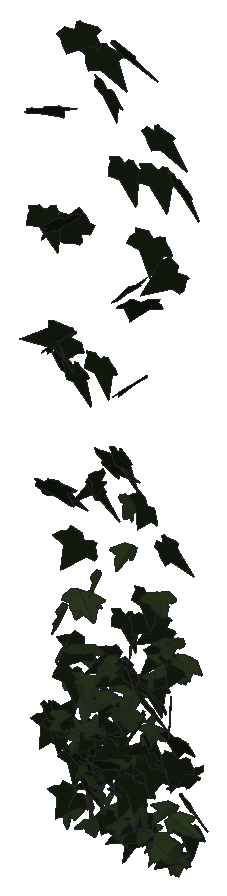
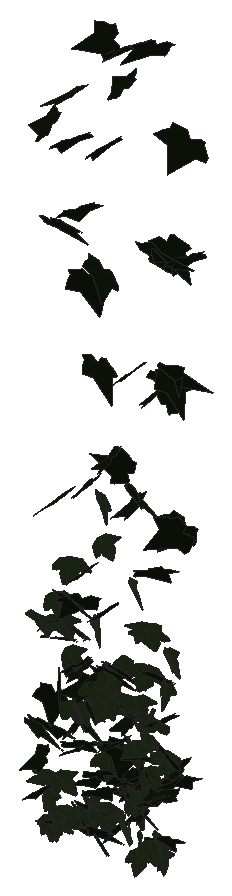
# SketchUp Ruby script. Lengths in inches.
U = 1.inch
M = Sketchup.active_model
def pt(a) = Geom::Point3d.new(a.map { |v| v * U })
def face(e, loops, mat)
  f = e.add_face(loops[0].map { |a| pt(a) })
  loops[1..].each { |l| e.add_face(l.map { |a| pt(a) }).erase! }
  f.material = f.back_material = mat if mat
  f
end
# faces: each face lists its corners as indices into pts; further lists are holes
def faces(e, pts, list, mat = nil) = list.each { |f| face(e, (f[0].is_a?(Array) ? f : [f]).map { |l| l.map { |i| pts[i] } }, mat) }
# xy, xz, yz: faces in a plane at the given z, y or x. An outline is a flat list of corners, or four numbers for a rectangle; further outlines are holes
def ring(l) = l.size == 4 ? [[l[0], l[1]], [l[2], l[1]], [l[2], l[3]], [l[0], l[3]]] : l.each_slice(2).to_a
def flat(e, list, mat, &to3) = list.each { |f| face(e, (f[0].is_a?(Array) ? f : [f]).map { |l| ring(l).map { |u, v| to3.(u, v) } }, mat) }
def xy(e, z, list, mat = nil) = flat(e, list, mat) { |x, y| [x, y, z] }
def xz(e, y, list, mat = nil) = flat(e, list, mat) { |x, z| [x, y, z] }
def yz(e, x, list, mat = nil) = flat(e, list, mat) { |y, z| [x, y, z] }
def lines(e, pts, list) = list.each { |a, b| e.add_line(pt(pts[a]), pt(pts[b])) }
# prism: a flat outline (further loops are holes) pulled along v
def prism(e, loops, v, mat = nil)
  f = face(e, loops, mat); d = Geom::Vector3d.new(v.map { |x| x * U })
  f.pushpull(f.normal.samedirection?(d) ? d.length : -d.length)
end
def box(e, o, s, mat = nil) = prism(e, [[o, [o[0] + s[0], o[1], o[2]], [o[0] + s[0], o[1] + s[1], o[2]], [o[0], o[1] + s[1], o[2]]]], [0, 0, s[2]], mat)
def at(x, y, z, deg = 0) = Geom::Transformation.translation(pt([x, y, z])) * Geom::Transformation.rotation(ORIGIN, Z_AXIS, deg.degrees)
def axes(o, x, y, z) = Geom::Transformation.new([*x, 0, *y, 0, *z, 0, *pt(o).to_a, 1])
def part(name) = M.definitions.add(name)
# library, detail: a bought-in or finely detailed component or shape, given as its bounding box
def library(name, o, s) = part(name).tap { |d| box(d.entities, o, s) }
def detail(e, o, s) = box(e.add_group.entities, o, s)
def put(e, d, t, mat = nil) = e.add_instance(d, t).tap { |i| i.material = mat if mat }
def group(e, t, mat = nil) = e.add_group.tap { |g| g.transformation = t; g.material = mat if mat }.entities
root = M.entities
M.materials.add("1026 AP 7946 SUNNY SIDE UP").color = [254, 231, 186]
M.materials.add("efeu1").color = [18, 25, 13]
M.materials.add("efeu2").color = [43, 57, 29]
c1 = part("ivyleaf_9")
p = [[1.54,2.16,1.25],[1.36,2.04,1.19],[-0.21,0.99,0.68],[-0.71,1.11,0.82],[-0.85,0.86,0.67],[-0.8,0.17,0.21],
  [-0.9,-0.01,0.1],[-0.67,-0.16,-0.02],[-0.08,-0.08,-0.05],[-0.03,-0.6,-0.4],[0.65,-0.88,-0.66],[0.83,-0.6,-0.49],
  [1.29,-0.42,-0.43],[1.8125,-0.07,-0.26],[1.21,0.44,0.15]]
faces(c1.entities,p,[[0,1,2,3,4,5,6,7,8,9,10,11,12,13,14]],"efeu1")
c2 = part("ivyleaf_10")
p = [[0,0.5,-0.03],[-0.0625,2.02,-0.43],[-0.19,2.01,-0.46],[-0.54,1.05,-0.29],[-0.52,0.625,-0.18],[-0.83,0.76,-0.28],
  [-1.16,0.64,-0.33],[-1.15,0.33,-0.24],[-0.77,-0.39,0.02],[-0.3,-0.51,0.16],[0.04,-0.48,0.23],[-0.02,2.01,-0.4375],
  [-0.06,2.01,-0.43],[0.04,-0.49,0.23],[0.67,-0.49,0.14],[1.38,0.36,-0.2],[1.375,0.51,-0.24],[0.81,0.65,-0.19],
  [0.62,0.59,-0.15],[0.6,1.09,-0.28],[0.5,1.23,-0.31]]
faces(c2.entities,p,[[0,1,2,3,4,5,6,7,8,9,10],[11,12,0,13,14,15,16,17,18,19,20]],"efeu2")
put(root,c1,axes([140.27,212.33,315.16],[-0.05103,-0.41878,-0.14855],[0.02164,0.14117,-0.43188],[0.69488,-0.03515,0.00254]),"1026 AP 7946 SUNNY SIDE UP")
put(root,c1,axes([140.4375,211.97,319.57],[0.50058,0.35673,0.06426],[-0.02996,0.0968,-0.4854],[-0.56811,0.30923,0.08221]),"1026 AP 7946 SUNNY SIDE UP")
put(root,c1,axes([140.57,212.51,294.58],[-0.36705,-0.28376,0.04945],[-0.02292,-0.05214,-0.37818],[0.45238,-0.23288,0.02096]),"1026 AP 7946 SUNNY SIDE UP")
put(root,c1,axes([140.3,212.48,295.11],[0.31532,-0.31436,-0.0618],[-0.04224,0.05189,-0.38379],[0.50093,0.20226,0.00653]),"1026 AP 7946 SUNNY SIDE UP")
put(root,c1,axes([140.9,212.33,310.2],[-0.0672,0.44029,-0.05517],[0.00492,-0.05601,-0.45604],[-0.69789,-0.04279,0.0021]),"1026 AP 7946 SUNNY SIDE UP")
put(root,c1,axes([141.19,212.43,310.375],[-0.10965,-0.09175,-0.44165],[-0.41434,-0.3375,0.11673],[-0.54994,0.27258,0.00011]),"1026 AP 7946 SUNNY SIDE UP")
put(root,c1,axes([140.54,212.12,304.4],[0.60737,0.11779,-0.0227],[-0.01672,-0.04262,-0.41446],[-0.18788,0.38458,-0.03649]),"1026 AP 7946 SUNNY SIDE UP")
put(root,c1,axes([140.66,212.67,294.48],[-0.12026,-0.35836,0.0457],[-0.00253,-0.04709,-0.37768],[0.56819,-0.07606,0.00799]),"1026 AP 7946 SUNNY SIDE UP")
put(root,c1,axes([140.51,212.26,304.2],[0.63153,0.08305,0.10577],[0.17132,-0.02531,-0.42006],[-0.1163,0.41366,-0.04441]),"1026 AP 7946 SUNNY SIDE UP")
put(root,c1,axes([141.07,212.35,309.2],[0.26067,-0.24492,0.33514],[-0.16241,0.31599,0.29988],[-0.62117,-0.1854,0.06224]),"1026 AP 7946 SUNNY SIDE UP")
put(root,c2,axes([140.95,212.3,299.18],[0.16917,-0.36964,0.06288],[0.00554,-0.06468,-0.3967],[0.58962,0.10666,-0.01431]),"1026 AP 7946 SUNNY SIDE UP")
put(root,c2,axes([140.92,212.49,299.25],[0.31682,-0.31954,0.1033],[0.04111,-0.10376,-0.38837],[0.52586,0.20063,-0.03187]),"1026 AP 7946 SUNNY SIDE UP")
put(root,c1,axes([141.22,212.12,315.29],[-0.08166,0.39451,-0.22855],[-0.01903,-0.22668,-0.40955],[-0.71317,-0.03912,0.0371]),"1026 AP 7946 SUNNY SIDE UP")
put(root,c1,axes([141.66,212.4375,314.79],[-0.23021,0.14305,0.4165],[-0.53671,0.21835,-0.20607],[-0.40626,-0.36953,0.03623]),"1026 AP 7946 SUNNY SIDE UP")
put(root,c1,axes([141,212.22,294.9],[-0.30917,0.27819,0.21651],[0.18946,-0.17027,0.34995],[0.51285,0.23061,0.00124]),"1026 AP 7946 SUNNY SIDE UP")
put(root,c2,axes([141.18,212.26,297.93],[0.00805,-0.35803,-0.18452],[0.06659,0.17658,-0.36551],[0.62452,-0.01421,0.04135]),"1026 AP 7946 SUNNY SIDE UP")
put(root,c2,axes([141.39,212.22,295.08],[0.47396,-0.01439,-0.23336],[-0.35019,0.05326,-0.30858],[0.06825,0.37322,0.03727]),"1026 AP 7946 SUNNY SIDE UP")
put(root,c2,axes([141.16,212.49,291.29],[-0.00569,-0.34874,0.06949],[0.12653,-0.06843,-0.3502],[0.54462,0.01226,0.08209]),"1026 AP 7946 SUNNY SIDE UP")
put(root,c1,axes([141.34,212.51,291.95],[-0.43317,-0.23152,0.01127],[0.01363,-0.0293,-0.36977],[0.3643,-0.2742,0.02723]),"1026 AP 7946 SUNNY SIDE UP")
put(root,c2,axes([141.32,212.64,292.03],[0.22658,-0.33741,-0.01255],[-0.00765,0.00908,-0.37792],[0.53074,0.14418,-0.00009]),"1026 AP 7946 SUNNY SIDE UP")
put(root,c2,axes([141.0625,212.53,295.0625],[0.30439,-0.2512,0.21366],[0.34212,-0.0819,-0.30976],[0.38312,0.27271,0.10687]),"1026 AP 7946 SUNNY SIDE UP")
put(root,c1,axes([141.15,212.66,296.77],[-0.07297,-0.37912,-0.02091],[0.03044,0.01589,-0.39298],[0.59603,-0.04723,0.01751]),"1026 AP 7946 SUNNY SIDE UP")
put(root,c1,axes([141.13,212.63,293.65],[-0.13427,-0.28959,0.21536],[0.31555,-0.21809,-0.22629],[0.46639,0.06418,0.2151]),"1026 AP 7946 SUNNY SIDE UP")
put(root,c2,axes([141.58,212.65,291.67],[-0.35002,-0.27086,0.09031],[-0.00772,-0.1095,-0.35581],[0.44834,-0.21335,0.06438]),"1026 AP 7946 SUNNY SIDE UP")
put(root,c1,axes([141.54,212.64,293.45],[-0.20851,-0.3427,0.05843],[0.0096,-0.06507,-0.37777],[0.54661,-0.12958,0.02892]),"1026 AP 7946 SUNNY SIDE UP")
put(root,c2,axes([141.75,212.54,294.4],[-0.15602,-0.31038,0.17899],[-0.03212,-0.17693,-0.33527],[0.55974,-0.09667,0.03065]),"1026 AP 7946 SUNNY SIDE UP")
put(root,c1,axes([141.79,212.46,302.34],[-0.46187,-0.29028,0.06023],[-0.03319,-0.06393,-0.42467],[0.46495,-0.29293,0.02952]),"1026 AP 7946 SUNNY SIDE UP")
put(root,c2,axes([141.38,212.6,296.58],[0.49346,0.11332,0.21476],[0.32955,0.02739,-0.34127],[-0.173,0.3754,-0.03752]),"1026 AP 7946 SUNNY SIDE UP")
put(root,c1,axes([141.89,212.37,298.23],[-0.59094,-0.10328,-0.02932],[0.06474,-0.04568,-0.3978],[0.15526,-0.37407,0.05429]),"1026 AP 7946 SUNNY SIDE UP")
put(root,c2,axes([141.64,212.61,300],[0.5861,0.1408,-0.03835],[-0.03035,-0.05581,-0.40816],[-0.22731,0.3705,-0.04438]),"1026 AP 7946 SUNNY SIDE UP")
put(root,c2,axes([141.82,212.27,296.57],[-0.20291,0.34701,0.07481],[-0.05385,0.06261,-0.3809],[-0.55422,-0.13313,0.00962]),"1026 AP 7946 SUNNY SIDE UP")
put(root,c1,axes([141.57,212.27,309.35],[0.23878,-0.40183,-0.02146],[-0.02673,0.0134,-0.44231],[0.63195,0.1524,-0.0106]),"1026 AP 7946 SUNNY SIDE UP")
put(root,c1,axes([141.6875,212.25,323.01],[0.1133,-0.29523,-0.36052],[0.0929,0.35565,-0.29591],[0.71188,0.00057,0.09599]),"1026 AP 7946 SUNNY SIDE UP")
put(root,c2,axes([141.92,212.48,295.92],[0.51465,-0.16428,0.11376],[0.14985,-0.05829,-0.3775],[0.27373,0.34078,-0.00722]),"1026 AP 7946 SUNNY SIDE UP")
put(root,c1,axes([142.32,212.25,294.15],[-0.01414,0.02527,0.41183],[-0.09221,0.39533,-0.0248],[-0.62283,-0.0591,-0.00568]),"1026 AP 7946 SUNNY SIDE UP")
put(root,c2,axes([141.88,212.375,300.09],[0.36462,0.31007,0.11714],[0.15168,0.06706,-0.39679],[-0.49567,0.24861,-0.03525]),"1026 AP 7946 SUNNY SIDE UP")
put(root,c2,axes([142.08,212.22,298.21],[-0.52991,-0.18021,-0.07781],[0.13377,-0.002,-0.39143],[0.27591,-0.34514,0.04032]),"1026 AP 7946 SUNNY SIDE UP")
put(root,c2,axes([142.14,212.5625,291.1],[-0.27695,-0.30984,-0.07147],[0.07114,0.052,-0.3666],[0.49356,-0.18135,0.01274]),"1026 AP 7946 SUNNY SIDE UP")
put(root,c2,axes([142.1,212.21,293.52],[0.00377,-0.33346,-0.1644],[0.09303,0.15599,-0.338],[0.57249,-0.02315,0.05601]),"1026 AP 7946 SUNNY SIDE UP")
put(root,c2,axes([142.15,212.5,291.67],[-0.22791,0.32533,-0.0754],[-0.05562,-0.09631,-0.36032],[-0.52203,-0.13177,0.07131]),"1026 AP 7946 SUNNY SIDE UP")
put(root,c1,axes([141.96,212.41,294.07],[0.26741,-0.32817,-0.01308],[-0.02667,0.0034,-0.3805],[0.5156,0.17038,-0.0129]),"1026 AP 7946 SUNNY SIDE UP")
put(root,c1,axes([142.32,212.6,294.83],[-0.40803,-0.26374,0.07918],[0.02976,-0.12457,-0.36809],[0.4316,-0.24075,0.10024]),"1026 AP 7946 SUNNY SIDE UP")
put(root,c1,axes([142.59,212.45,293.04],[-0.45307,0.227,-0.02686],[0.00491,-0.0401,-0.3769],[-0.35949,-0.28664,0.0287]),"1026 AP 7946 SUNNY SIDE UP")
put(root,c1,axes([142.03,212.32,292.83],[0.40398,-0.30202,-0.04531],[-0.07259,0.01612,-0.40761],[0.474,0.25987,-0.0238]),"1026 AP 7946 SUNNY SIDE UP")
put(root,c2,axes([142.61,212.21,292.79],[-0.47002,0.12116,0.23185],[-0.35052,0.04369,-0.33],[-0.19467,-0.3712,0.0344]),"1026 AP 7946 SUNNY SIDE UP")
put(root,c2,axes([142.39,212.41,296.95],[-0.30169,-0.31803,0.106],[0.0274,-0.12999,-0.37464],[0.52576,-0.17572,0.08035]),"1026 AP 7946 SUNNY SIDE UP")
put(root,c2,axes([142.4,212.55,293.3],[-0.52141,0.15638,-0.01607],[0.00175,-0.03614,-0.37645],[-0.24725,-0.33004,0.03122]),"1026 AP 7946 SUNNY SIDE UP")
put(root,c2,axes([142.47,212.37,295.125],[-0.29512,-0.33445,0.07364],[0.01329,-0.08818,-0.39229],[0.53823,-0.1812,0.05006]),"1026 AP 7946 SUNNY SIDE UP")
put(root,c1,axes([142.71,212.3125,305.17],[-0.5278,0.19491,-0.14126],[0.14523,-0.11399,-0.39732],[-0.34652,-0.34465,0.04864]),"1026 AP 7946 SUNNY SIDE UP")
put(root,c1,axes([142.48,212.73,293.9375],[-0.20009,-0.33888,0.08114],[-0.0045,-0.08488,-0.37241],[0.54774,-0.12449,0.02658]),"1026 AP 7946 SUNNY SIDE UP")
put(root,c2,axes([142.41,212.71,293.64],[0.41764,-0.21258,0.15038],[0.17783,-0.09422,-0.35102],[0.3656,0.28867,-0.00105]),"1026 AP 7946 SUNNY SIDE UP")
put(root,c2,axes([142.3,212.55,295.09],[-0.05262,-0.06988,-0.37603],[0.3321,-0.30466,0.0384],[-0.48008,-0.20309,0.06778]),"1026 AP 7946 SUNNY SIDE UP")
put(root,c2,axes([142.65,212.23,301.29],[0.30959,-0.34036,0.05782],[0.01384,-0.06186,-0.40474],[0.54273,0.19573,-0.02266]),"1026 AP 7946 SUNNY SIDE UP")
put(root,c1,axes([142.34,212.46,304.79],[0.39666,-0.32966,-0.06343],[-0.0382,0.05654,-0.42703],[0.5254,0.25299,0.01684]),"1026 AP 7946 SUNNY SIDE UP")
put(root,c2,axes([142.48,212.71,291.8],[0.00206,0.04334,0.38202],[0.36753,-0.28895,0.03227],[0.45728,0.23204,-0.02766]),"1026 AP 7946 SUNNY SIDE UP")
put(root,c1,axes([142.88,212.24,293.89],[0.28202,0.21252,-0.2683],[-0.24237,-0.21187,-0.28738],[-0.47137,0.23609,-0.01276]),"1026 AP 7946 SUNNY SIDE UP")
put(root,c1,axes([142.45,212.6,296.26],[0.35817,-0.29911,0.01108],[-0.00512,-0.01813,-0.38717],[0.47069,0.2274,-0.01265]),"1026 AP 7946 SUNNY SIDE UP")
put(root,c1,axes([143.19,212.39,293.68],[-0.52388,0.13029,0.09975],[-0.16367,-0.00404,-0.36623],[-0.19495,-0.34673,0.03943]),"1026 AP 7946 SUNNY SIDE UP")
put(root,c1,axes([142.59,212.48,309.89],[0.06045,-0.42323,0.02377],[-0.00982,-0.02614,-0.43786],[0.66662,0.03799,-0.0086]),"1026 AP 7946 SUNNY SIDE UP")
put(root,c1,axes([142.48,212.45,293.49],[0.29359,-0.31008,0.0621],[0.10526,-0.03166,-0.37073],[0.48596,0.19419,0.04278]),"1026 AP 7946 SUNNY SIDE UP")
put(root,c1,axes([142.92,212.36,294.92],[0.32698,0.30252,-0.05125],[-0.08375,-0.02565,-0.37715],[-0.4752,0.21268,0.0312]),"1026 AP 7946 SUNNY SIDE UP")
put(root,c2,axes([142.9,212.62,292.2],[0.242,-0.32997,0.03861],[0.00989,-0.04046,-0.37514],[0.52242,0.15362,-0.01078]),"1026 AP 7946 SUNNY SIDE UP")
put(root,c1,axes([143.28,212.58,298.07],[-0.5928,0.04064,0.00855],[-0.02164,-0.05317,-0.38692],[-0.06145,-0.37332,0.05378]),"1026 AP 7946 SUNNY SIDE UP")
put(root,c2,axes([143.27,212.3,296.61],[-0.32524,-0.21297,0.24871],[-0.23033,-0.19488,-0.30601],[0.45238,-0.25234,0.02301]),"1026 AP 7946 SUNNY SIDE UP")
put(root,c1,axes([143.1,212.36,296.53],[-0.47864,0.00761,-0.23912],[0.36193,-0.04151,-0.31256],[-0.04904,-0.38057,0.02705]),"1026 AP 7946 SUNNY SIDE UP")
put(root,c1,axes([142.79,212.23,322.56],[0.14553,-0.40252,-0.20127],[0.09161,0.2064,-0.41328],[0.69598,0.057,0.09648]),"1026 AP 7946 SUNNY SIDE UP")
put(root,c1,axes([142.92,212.47,320.97],[0.08303,-0.37541,0.25931],[0.10464,-0.24636,-0.39105],[0.70485,0.0808,0.02751]),"1026 AP 7946 SUNNY SIDE UP")
put(root,c1,axes([143.03,212.68,295.24],[0.10232,-0.35605,-0.11245],[0.01303,0.11013,-0.3712],[0.5845,0.05987,0.02796]),"1026 AP 7946 SUNNY SIDE UP")
put(root,c1,axes([142.79,212.51,305.91],[0.31432,-0.15126,0.34045],[0.36694,-0.23699,-0.25789],[0.4397,0.3059,-0.02815]),"1026 AP 7946 SUNNY SIDE UP")
put(root,c1,axes([143.11,212.2,291.81],[0.21127,-0.3081,-0.21836],[-0.09772,0.20182,-0.34447],[0.57828,0.14667,0.02156]),"1026 AP 7946 SUNNY SIDE UP")
put(root,c2,axes([143.22,212.01,298.05],[-0.11799,-0.27684,-0.27266],[0.2331,0.22599,-0.28721],[0.55344,-0.1542,0.06284]),"1026 AP 7946 SUNNY SIDE UP")
put(root,c1,axes([143.72,212.42,294.79],[-0.57897,-0.06393,0.06447],[-0.08978,-0.03809,-0.38419],[0.10881,-0.3716,0.02602]),"1026 AP 7946 SUNNY SIDE UP")
put(root,c2,axes([143.54,212.5,297.65],[-0.21234,-0.34751,0.15485],[-0.00704,-0.16018,-0.38157],[0.59655,-0.12559,0.05062]),"1026 AP 7946 SUNNY SIDE UP")
put(root,c2,axes([143.59,212.5,294.32],[-0.49677,-0.19025,0.02433],[-0.0104,-0.03675,-0.37904],[0.30149,-0.31475,0.02701]),"1026 AP 7946 SUNNY SIDE UP")
put(root,c1,axes([143.83,212.52,297.76],[-0.60292,-0.03012,0.05267],[-0.07593,-0.0378,-0.39494],[0.05462,-0.385,0.03237]),"1026 AP 7946 SUNNY SIDE UP")
put(root,c1,axes([143.31,212.66,306.31],[0.28624,-0.37058,0.00439],[-0.02322,-0.01433,-0.42494],[0.58232,0.18158,-0.0191]),"1026 AP 7946 SUNNY SIDE UP")
put(root,c2,axes([143.78,212.49,292.28],[-0.36455,-0.27079,0.08077],[-0.05524,-0.07497,-0.36701],[0.44051,-0.2335,0.02082]),"1026 AP 7946 SUNNY SIDE UP")
put(root,c2,axes([143.8,212.51,296.5],[-0.21829,-0.30662,0.18687],[-0.04272,-0.18684,-0.3446],[0.55995,-0.13379,0.04656]),"1026 AP 7946 SUNNY SIDE UP")
put(root,c1,axes([143.83,212.75,293.8],[-0.42979,-0.24653,0.01811],[0.00846,-0.03421,-0.37822],[0.38869,-0.27185,0.02825]),"1026 AP 7946 SUNNY SIDE UP")
put(root,c2,axes([143.83,212.53,304.53],[0.41947,-0.26278,-0.14687],[-0.07922,0.14685,-0.37908],[0.46223,0.26363,0.06831]),"1026 AP 7946 SUNNY SIDE UP")
put(root,c2,axes([143.85,212.45,302.74],[-0.19,-0.32236,0.21022],[0.02496,-0.21996,-0.34648],[0.60093,-0.09279,0.08086]),"1026 AP 7946 SUNNY SIDE UP")
put(root,c1,axes([143.34,212.6,322.78],[0.63705,-0.18433,0.1015],[0.13093,-0.05725,-0.45854],[0.30229,0.41325,-0.0153]),"1026 AP 7946 SUNNY SIDE UP")
put(root,c2,axes([143.92,212.17,291.78],[-0.27871,-0.31146,0.02248],[0.00323,-0.02829,-0.369],[0.49114,-0.17656,0.01518]),"1026 AP 7946 SUNNY SIDE UP")
put(root,c1,axes([144.04,212.19,313.28],[0.06669,0.40847,0.21459],[-0.02378,0.20801,-0.42051],[-0.71893,0.03101,0.03381]),"1026 AP 7946 SUNNY SIDE UP")
put(root,c1,axes([144.18,212.72,291.42],[-0.54974,-0.08522,0.10292],[-0.13151,-0.07628,-0.36723],[0.15992,-0.35565,0.0518]),"1026 AP 7946 SUNNY SIDE UP")
put(root,c1,axes([144.17,212.26,309.58],[-0.08678,0.44125,-0.03346],[-0.00126,-0.03536,-0.45829],[-0.696,-0.05495,0.005]),"1026 AP 7946 SUNNY SIDE UP")
put(root,c2,axes([143.98,212.65,297.08],[-0.46785,-0.24019,0.03416],[0.06334,-0.10275,-0.37945],[0.37627,-0.28136,0.10634]),"1026 AP 7946 SUNNY SIDE UP")
put(root,c1,axes([144.02,212.55,292.9375],[-0.36105,-0.28347,0.0414],[-0.01371,-0.04663,-0.37538],[0.45034,-0.22869,0.02177]),"1026 AP 7946 SUNNY SIDE UP")
put(root,c2,axes([144.01,212.17,296.3],[-0.58726,-0.11529,-0.05292],[0.08662,-0.00679,-0.40204],[0.1781,-0.37685,0.02102]),"1026 AP 7946 SUNNY SIDE UP")
put(root,c1,axes([143.8,212.39,300.03],[0.0725,-0.39174,-0.04245],[-0.0146,0.03815,-0.4061],[0.61884,0.04679,-0.00461]),"1026 AP 7946 SUNNY SIDE UP")
put(root,c1,axes([144.02,212.625,291.21],[-0.43444,0.05657,-0.23965],[0.34731,-0.07803,-0.28987],[-0.14646,-0.35286,0.02346]),"1026 AP 7946 SUNNY SIDE UP")
put(root,c1,axes([143.83,212.33,318.3],[0.05309,-0.44977,-0.05448],[-0.01708,0.04965,-0.46431],[0.71143,0.03476,-0.00708]),"1026 AP 7946 SUNNY SIDE UP")
put(root,c1,axes([143.81,212.65,297.65],[0.22168,-0.35751,0.03918],[0.00065,-0.04287,-0.39584],[0.56567,0.14016,-0.0149]),"1026 AP 7946 SUNNY SIDE UP")
put(root,c2,axes([144.35,212.09,299.21],[-0.02427,0.24732,0.30292],[-0.3718,0.2243,-0.20683],[-0.47406,-0.18858,0.14671]),"1026 AP 7946 SUNNY SIDE UP")
put(root,c1,axes([144.42,212.58,292.21],[-0.55784,-0.07015,-0.06047],[0.10708,-0.04795,-0.36776],[0.09541,-0.35631,0.05919]),"1026 AP 7946 SUNNY SIDE UP")
put(root,c1,axes([144.46,212.39,312.95],[0.18934,0.36354,-0.19677],[-0.1076,-0.18068,-0.39551],[-0.63824,0.13831,0.0083]),"1026 AP 7946 SUNNY SIDE UP")
put(root,c1,axes([144.26,212.58,293.33],[-0.23225,-0.33893,0.00795],[0.01693,-0.0152,-0.38062],[0.53288,-0.14724,0.01555]),"1026 AP 7946 SUNNY SIDE UP")
put(root,c2,axes([144.3,212.33,292.46],[0.00522,-0.36165,0.10964],[0.18094,-0.10236,-0.35575],[0.56544,0.03609,0.11283]),"1026 AP 7946 SUNNY SIDE UP")
put(root,c1,axes([144.52,212.39,296.17],[-0.34987,0.11574,-0.28647],[0.33354,-0.18635,-0.25526],[-0.33757,-0.30409,0.04469]),"1026 AP 7946 SUNNY SIDE UP")
put(root,c2,axes([144.56,212.41,292.33],[0.40145,-0.27372,-0.04448],[-0.0013,0.05587,-0.38336],[0.43535,0.25257,0.03988]),"1026 AP 7946 SUNNY SIDE UP")
put(root,c1,axes([144.95,212.25,295.34],[-0.42289,0.26087,-0.03618],[0.01046,-0.04557,-0.38518],[-0.41407,-0.26757,0.02722]),"1026 AP 7946 SUNNY SIDE UP")
put(root,c1,axes([144.55,212.64,304.66],[-0.11579,-0.31367,0.27731],[-0.04597,-0.27059,-0.33246],[0.65014,-0.075,0.02588]),"1026 AP 7946 SUNNY SIDE UP")
put(root,c1,axes([144.8,212.78,294.66],[-0.4533,-0.22659,0.06225],[-0.02348,-0.07982,-0.37428],[0.36852,-0.28381,0.05272]),"1026 AP 7946 SUNNY SIDE UP")
put(root,c2,axes([144.8,212.625,295.92],[0.2808,-0.33678,-0.00733],[0.00314,0.00695,-0.39263],[0.5296,0.17852,0.00621]),"1026 AP 7946 SUNNY SIDE UP")
put(root,c1,axes([144.6875,212.63,291.79],[-0.26257,-0.02106,-0.33712],[0.50255,-0.09199,-0.16252],[-0.11446,-0.35557,0.05978]),"1026 AP 7946 SUNNY SIDE UP")
put(root,c1,axes([144.5,212.53,296.79],[0.40291,-0.28203,0.07181],[0.07894,-0.05072,-0.39284],[0.45055,0.2611,0.00462]),"1026 AP 7946 SUNNY SIDE UP")
put(root,c2,axes([145.14,212.48,295.84],[-0.39169,-0.22242,0.18802],[-0.17737,-0.14839,-0.3434],[0.41756,-0.27168,0.03051]),"1026 AP 7946 SUNNY SIDE UP")
put(root,c1,axes([144.59,212.66,297.52],[0.21571,-0.3477,0.09692],[0.10031,-0.07776,-0.38429],[0.55826,0.14832,0.0316]),"1026 AP 7946 SUNNY SIDE UP")
put(root,c1,axes([144.71,212.53,300.25],[-0.06297,-0.2753,-0.31082],[0.10318,0.29329,-0.28444],[0.63204,-0.07531,0.01547]),"1026 AP 7946 SUNNY SIDE UP")
put(root,c2,axes([144.8125,212.375,291.69],[-0.23264,-0.22355,-0.27499],[0.29144,0.19334,-0.27281],[0.46166,-0.23471,0.03365]),"1026 AP 7946 SUNNY SIDE UP")
put(root,c1,axes([144.78,212.41,301.18],[0.00918,-0.39588,0.06446],[-0.02008,-0.06498,-0.40802],[0.63045,0.00369,-0.01393]),"1026 AP 7946 SUNNY SIDE UP")
put(root,c1,axes([144.78,212.47,295.46],[0.34501,-0.27536,-0.13154],[-0.16081,0.07922,-0.36104],[0.44825,0.24036,-0.02828]),"1026 AP 7946 SUNNY SIDE UP")
put(root,c1,axes([144.87,212.5625,315.56],[-0.21714,-0.4199,-0.01131],[0.01645,0.0056,-0.45526],[0.66019,-0.13825,0.00762]),"1026 AP 7946 SUNNY SIDE UP")
put(root,c2,axes([145.1,212.67,298.03],[-0.11733,-0.34754,0.15386],[0.00113,-0.15436,-0.36575],[0.59602,-0.06812,0.03098]),"1026 AP 7946 SUNNY SIDE UP")
put(root,c1,axes([144.86,212.6,297.63],[-0.00559,-0.37529,-0.07194],[0.0142,0.0676,-0.38615],[0.59947,-0.0051,0.00848]),"1026 AP 7946 SUNNY SIDE UP")
put(root,c1,axes([145,212.55,294.24],[-0.1757,-0.34341,0.09742],[0.02056,-0.10501,-0.36995],[0.56052,-0.10379,0.04411]),"1026 AP 7946 SUNNY SIDE UP")
put(root,c1,axes([145.49,212.53,300.09],[-0.6033,0.06037,-0.01314],[0.01091,-0.03977,-0.39842],[-0.09652,-0.38184,0.0371]),"1026 AP 7946 SUNNY SIDE UP")
put(root,c2,axes([145.45,212.62,291.46],[-0.18571,-0.16924,0.31025],[-0.18191,-0.28158,-0.21073],[0.51322,-0.16105,0.03757]),"1026 AP 7946 SUNNY SIDE UP")
put(root,c1,axes([145.03,212.66,318.3],[-0.05994,-0.44003,-0.08041],[0.04667,0.07316,-0.45397],[0.70048,-0.04253,0.02337]),"1026 AP 7946 SUNNY SIDE UP")
put(root,c1,axes([145.41,212.54,299.12],[-0.5629,0.01304,-0.1693],[0.23437,-0.14263,-0.34683],[-0.11103,-0.36721,0.12623]),"1026 AP 7946 SUNNY SIDE UP")
put(root,c2,axes([145.3125,212.35,301.39],[-0.44164,-0.27988,-0.06139],[0.16356,-0.02435,-0.39803],[0.41861,-0.28576,0.09075]),"1026 AP 7946 SUNNY SIDE UP")
put(root,c2,axes([145.375,212.35,291.29],[-0.00009,-0.26974,0.26394],[0.08183,-0.25522,-0.27665],[0.58089,0.03591,0.03901]),"1026 AP 7946 SUNNY SIDE UP")
put(root,c2,axes([145.61,212.58,292.88],[-0.16929,-0.28698,0.24515],[-0.08293,-0.23518,-0.31598],[0.58196,-0.117,0.02628]),"1026 AP 7946 SUNNY SIDE UP")
put(root,c1,axes([145.11,212.48,319.99],[0.32578,-0.38963,-0.11622],[0.06679,0.14445,-0.44142],[0.63336,0.18518,0.10633]),"1026 AP 7946 SUNNY SIDE UP")
put(root,c1,axes([145.68,212.73,298.49],[-0.48594,-0.22787,0.04439],[0.08036,-0.13886,-0.36868],[0.35608,-0.27963,0.14378]),"1026 AP 7946 SUNNY SIDE UP")
put(root,c2,axes([145.86,212.35,298.97],[-0.44975,-0.18081,0.18916],[-0.15894,-0.17521,-0.33908],[0.37398,-0.2919,0.08338]),"1026 AP 7946 SUNNY SIDE UP")
put(root,c1,axes([145.98,212.44,314.65],[-0.67957,-0.04238,0.00177],[0.0038,-0.04458,-0.44526],[0.0666,-0.42988,0.04344]),"1026 AP 7946 SUNNY SIDE UP")
put(root,c1,axes([145.84,212.3,296.2],[-0.00752,-0.05621,0.40887],[0.08785,0.39327,0.06033],[-0.62464,0.05598,0.00356]),"1026 AP 7946 SUNNY SIDE UP")
put(root,c2,axes([145.52,212.15,291.42],[0.23836,0.27888,0.24565],[0.13172,0.22312,-0.32456],[-0.56005,0.17117,0.02821]),"1026 AP 7946 SUNNY SIDE UP")
put(root,c2,axes([145.93,212.35,299.78],[-0.31482,-0.33395,0.05665],[-0.0162,-0.06004,-0.40085],[0.53243,-0.19929,0.0213]),"1026 AP 7946 SUNNY SIDE UP")
put(root,c1,axes([145.99,212.75,291.13],[-0.4651,-0.16606,0.10116],[-0.05337,-0.13378,-0.33595],[0.29939,-0.28182,0.09727]),"1026 AP 7946 SUNNY SIDE UP")
put(root,c2,axes([145.95,212.4375,291.01],[-0.54133,-0.07848,-0.0136],[0.03207,-0.03238,-0.36205],[0.12084,-0.34298,0.03516]),"1026 AP 7946 SUNNY SIDE UP")
put(root,c2,axes([146.14,212.56,290.99],[-0.16032,-0.31923,0.10621],[-0.05317,-0.09933,-0.34581],[0.52569,-0.1074,-0.00259]),"1026 AP 7946 SUNNY SIDE UP")
put(root,c1,axes([146.09,212.29,295.9375],[0.47242,0.06561,-0.23429],[-0.3444,-0.06383,-0.31692],[-0.14257,0.37159,-0.01077]),"1026 AP 7946 SUNNY SIDE UP")
put(root,c1,axes([146.01,212.61,294.87],[-0.45966,-0.16097,-0.17466],[0.29163,0.00327,-0.33443],[0.22208,-0.33747,0.07765]),"1026 AP 7946 SUNNY SIDE UP")
put(root,c1,axes([145.81,212.1,303.77],[0.36663,-0.28906,-0.21575],[-0.08818,0.21545,-0.37236],[0.55277,0.22609,0.08369]),"1026 AP 7946 SUNNY SIDE UP")
put(root,c1,axes([146.03,212.56,298.84],[-0.19089,-0.32347,0.17344],[-0.03664,-0.17212,-0.35514],[0.57356,-0.11865,0.03503]),"1026 AP 7946 SUNNY SIDE UP")
put(root,c2,axes([146.42,212.21,291.7],[0.02077,-0.38611,0.00395],[0.00596,-0.0059,-0.39801],[0.60716,0.01327,0.00377]),"1026 AP 7946 SUNNY SIDE UP")
put(root,c2,axes([146.36,212.66,298.98],[0.60914,-0.05653,0.00383],[-0.00244,-0.03846,-0.40161],[0.08908,0.3855,-0.03718]),"1026 AP 7946 SUNNY SIDE UP")
put(root,c2,axes([146.16,212.32,292.65],[-0.28846,-0.15506,-0.29029],[0.48994,-0.00889,-0.20464],[0.12039,-0.33538,0.13725]),"1026 AP 7946 SUNNY SIDE UP")
put(root,c1,axes([146.39,212.78,292.2],[-0.05794,-0.36027,0.02078],[-0.00593,-0.02195,-0.37321],[0.56753,-0.03701,-0.00178]),"1026 AP 7946 SUNNY SIDE UP")
put(root,c1,axes([146.17,212.43,318.36],[0.30878,-0.3763,0.15279],[0.06988,-0.14618,-0.43727],[0.63339,0.19958,-0.02624]),"1026 AP 7946 SUNNY SIDE UP")
put(root,c1,axes([146.89,212.49,294.62],[-0.43658,0.23965,-0.07783],[0.00283,-0.11262,-0.36887],[-0.39574,-0.26519,0.08322]),"1026 AP 7946 SUNNY SIDE UP")
put(root,c1,axes([146.35,212.54,293.45],[0.43587,-0.24876,-0.01544],[-0.04103,-0.00879,-0.38295],[0.38957,0.27739,-0.02306]),"1026 AP 7946 SUNNY SIDE UP")
